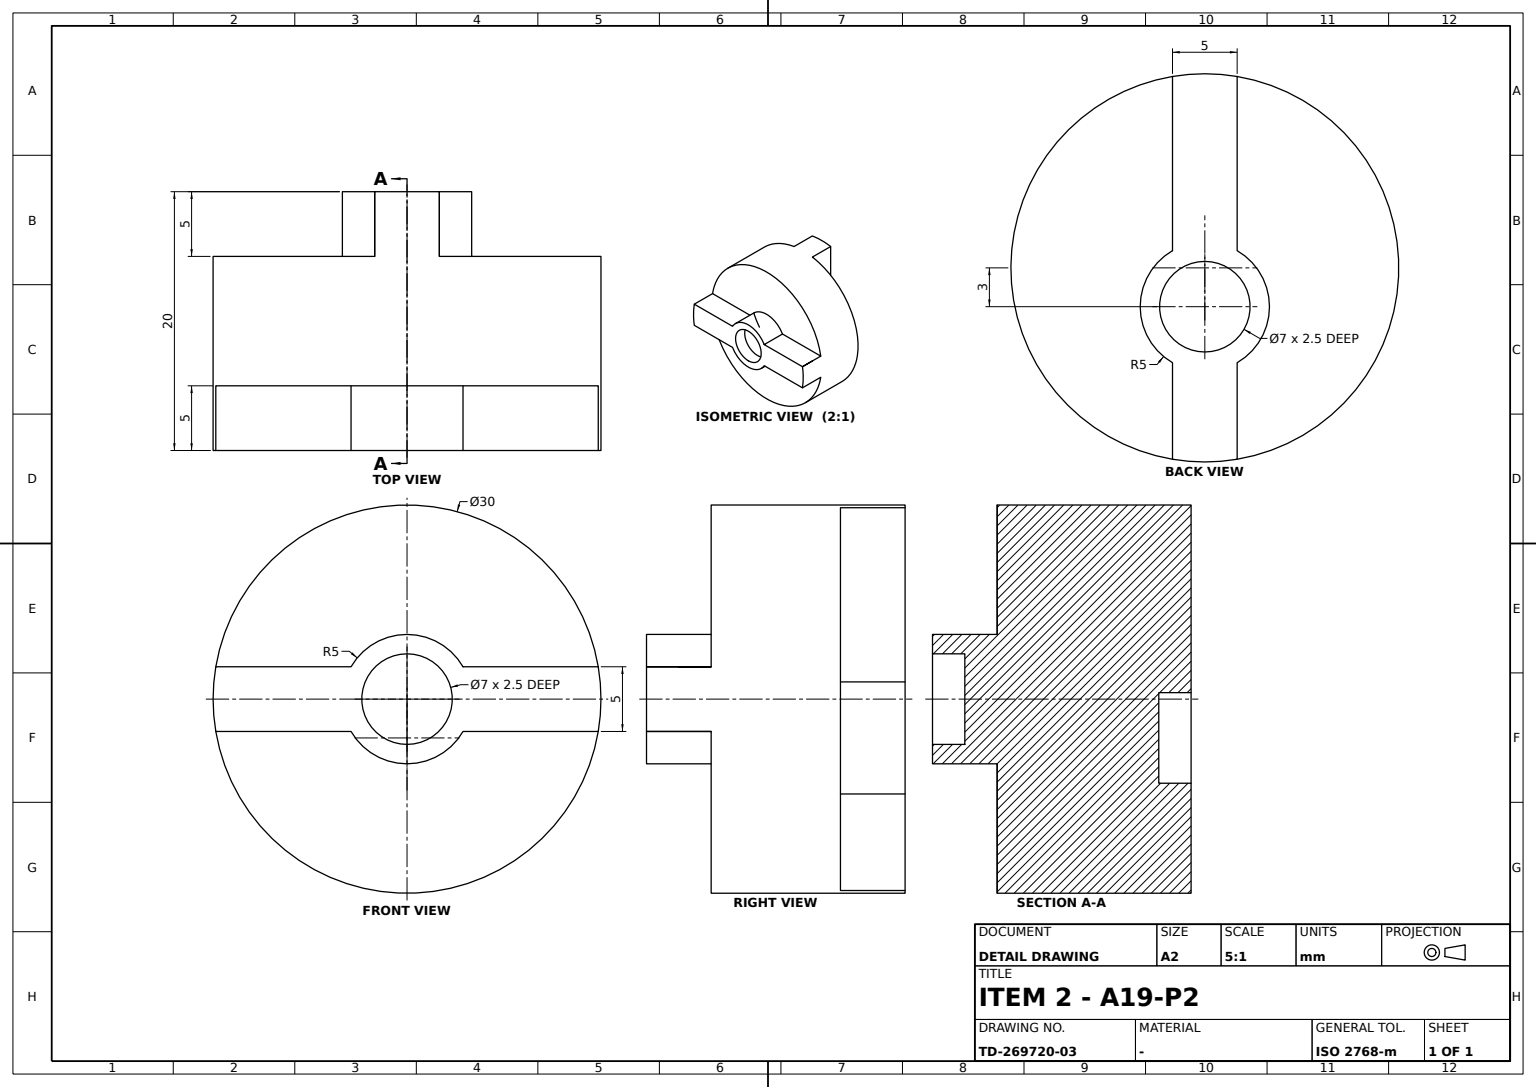
ISO-10303-21;
HEADER;
FILE_DESCRIPTION((''),'2;1');
FILE_NAME('','',(''),(''),'','','');
FILE_SCHEMA(('AUTOMOTIVE_DESIGN'));
ENDSEC;
DATA;
#1=APPLICATION_CONTEXT('');
#2=PRODUCT_CONTEXT('',#1,'mechanical');
#3=PRODUCT('','','',(#2));
#4=PRODUCT_DEFINITION_FORMATION('','',#3);
#5=PRODUCT_DEFINITION_CONTEXT('',#1,'design');
#6=PRODUCT_DEFINITION('','',#4,#5);
#7=PRODUCT_DEFINITION_SHAPE('','',#6);
#8=(LENGTH_UNIT()NAMED_UNIT(*)SI_UNIT(.MILLI.,.METRE.));
#9=(NAMED_UNIT(*)PLANE_ANGLE_UNIT()SI_UNIT($,.RADIAN.));
#10=(NAMED_UNIT(*)SI_UNIT($,.STERADIAN.)SOLID_ANGLE_UNIT());
#11=UNCERTAINTY_MEASURE_WITH_UNIT(LENGTH_MEASURE(0.005),#8,'distance_accuracy_value','');
#12=(GEOMETRIC_REPRESENTATION_CONTEXT(3)GLOBAL_UNCERTAINTY_ASSIGNED_CONTEXT((#11))GLOBAL_UNIT_ASSIGNED_CONTEXT((#8,#9,#10))REPRESENTATION_CONTEXT('',''));
#13=CARTESIAN_POINT('',(-7.5,0.,0.5));
#14=VERTEX_POINT('',#13);
#15=CARTESIAN_POINT('',(-7.5,0.,-3.));
#16=DIRECTION('',(-1.,0.,0.));
#17=DIRECTION('',(0.,0.,1.));
#18=AXIS2_PLACEMENT_3D('',#15,#16,#17);
#19=CIRCLE('',#18,3.5);
#20=EDGE_CURVE('',#14,#14,#19,.T.);
#21=ORIENTED_EDGE('',*,*,#20,.F.);
#22=EDGE_LOOP('',(#21));
#23=FACE_BOUND('',#22,.T.);
#24=CARTESIAN_POINT('',(-10.,0.,0.5));
#25=VERTEX_POINT('',#24);
#26=CARTESIAN_POINT('',(-10.,0.,-3.));
#27=AXIS2_PLACEMENT_3D('',#26,#16,#17);
#28=CIRCLE('',#27,3.5);
#29=EDGE_CURVE('',#25,#25,#28,.T.);
#30=ORIENTED_EDGE('',*,*,#29,.T.);
#31=EDGE_LOOP('',(#30));
#32=FACE_BOUND('',#31,.T.);
#33=CARTESIAN_POINT('',(-8.75,0.,-3.));
#34=DIRECTION('',(0.,-1.,0.));
#35=AXIS2_PLACEMENT_3D('',#33,#16,#34);
#36=CYLINDRICAL_SURFACE('',#35,3.5);
#37=ADVANCED_FACE('',(#23,#32),#36,.F.);
#38=CARTESIAN_POINT('',(7.5,0.,-3.5));
#39=VERTEX_POINT('',#38);
#40=CARTESIAN_POINT('',(7.5,0.,0.));
#41=DIRECTION('',(1.,0.,0.));
#42=DIRECTION('',(0.,0.,-1.));
#43=AXIS2_PLACEMENT_3D('',#40,#41,#42);
#44=CIRCLE('',#43,3.5);
#45=EDGE_CURVE('',#39,#39,#44,.T.);
#46=ORIENTED_EDGE('',*,*,#45,.F.);
#47=EDGE_LOOP('',(#46));
#48=FACE_BOUND('',#47,.T.);
#49=CARTESIAN_POINT('',(10.,0.,-3.5));
#50=VERTEX_POINT('',#49);
#51=CARTESIAN_POINT('',(10.,0.,0.));
#52=AXIS2_PLACEMENT_3D('',#51,#41,#42);
#53=CIRCLE('',#52,3.5);
#54=EDGE_CURVE('',#50,#50,#53,.T.);
#55=ORIENTED_EDGE('',*,*,#54,.T.);
#56=EDGE_LOOP('',(#55));
#57=FACE_BOUND('',#56,.T.);
#58=CARTESIAN_POINT('',(8.75,0.,0.));
#59=DIRECTION('',(0.,1.,0.));
#60=AXIS2_PLACEMENT_3D('',#58,#41,#59);
#61=CYLINDRICAL_SURFACE('',#60,3.5);
#62=ADVANCED_FACE('',(#48,#57),#61,.F.);
#63=CARTESIAN_POINT('',(-5.,-2.5,1.330127));
#64=VERTEX_POINT('',#63);
#65=CARTESIAN_POINT('',(-10.,-2.5,1.330127));
#66=VERTEX_POINT('',#65);
#67=VECTOR('',#16,1000.);
#68=LINE('',#63,#67);
#69=EDGE_CURVE('',#64,#66,#68,.T.);
#70=ORIENTED_EDGE('',*,*,#69,.F.);
#71=CARTESIAN_POINT('',(-5.,-2.5,14.790199));
#72=VERTEX_POINT('',#71);
#73=CARTESIAN_POINT('',(-5.,-2.5,-7.330127));
#74=VECTOR('',#42,1000.);
#75=LINE('',#73,#74);
#76=EDGE_CURVE('',#72,#64,#75,.T.);
#77=ORIENTED_EDGE('',*,*,#76,.F.);
#78=CARTESIAN_POINT('',(-10.,-2.5,14.790199));
#79=VERTEX_POINT('',#78);
#80=VECTOR('',#41,1000.);
#81=LINE('',#71,#80);
#82=EDGE_CURVE('',#72,#79,#81,.F.);
#83=ORIENTED_EDGE('',*,*,#82,.T.);
#84=CARTESIAN_POINT('',(-10.,-2.5,0.));
#85=LINE('',#84,#74);
#86=EDGE_CURVE('',#79,#66,#85,.T.);
#87=ORIENTED_EDGE('',*,*,#86,.T.);
#88=EDGE_LOOP('',(#70,#77,#83,#87));
#89=FACE_BOUND('',#88,.T.);
#90=AXIS2_PLACEMENT_3D('',#73,#59,#42);
#91=PLANE('',#90);
#92=ADVANCED_FACE('',(#89),#91,.F.);
#93=CARTESIAN_POINT('',(-10.,2.5,14.790199));
#94=VERTEX_POINT('',#93);
#95=CARTESIAN_POINT('',(-10.,0.,0.));
#96=AXIS2_PLACEMENT_3D('',#95,#16,#17);
#97=CIRCLE('',#96,15.);
#98=EDGE_CURVE('',#79,#94,#97,.T.);
#99=ORIENTED_EDGE('',*,*,#98,.T.);
#100=CARTESIAN_POINT('',(-10.,2.5,1.330127));
#101=VERTEX_POINT('',#100);
#102=CARTESIAN_POINT('',(-10.,2.5,0.));
#103=VECTOR('',#17,1000.);
#104=LINE('',#102,#103);
#105=EDGE_CURVE('',#101,#94,#104,.T.);
#106=ORIENTED_EDGE('',*,*,#105,.F.);
#107=CARTESIAN_POINT('',(-10.,2.5,-7.330127));
#108=VERTEX_POINT('',#107);
#109=CIRCLE('',#27,5.);
#110=EDGE_CURVE('',#101,#108,#109,.T.);
#111=ORIENTED_EDGE('',*,*,#110,.T.);
#112=CARTESIAN_POINT('',(-10.,2.5,-14.790199));
#113=VERTEX_POINT('',#112);
#114=EDGE_CURVE('',#113,#108,#104,.T.);
#115=ORIENTED_EDGE('',*,*,#114,.F.);
#116=CARTESIAN_POINT('',(-10.,-2.5,-14.790199));
#117=VERTEX_POINT('',#116);
#118=EDGE_CURVE('',#113,#117,#97,.T.);
#119=ORIENTED_EDGE('',*,*,#118,.T.);
#120=CARTESIAN_POINT('',(-10.,-2.5,-7.330127));
#121=VERTEX_POINT('',#120);
#122=EDGE_CURVE('',#121,#117,#85,.T.);
#123=ORIENTED_EDGE('',*,*,#122,.F.);
#124=EDGE_CURVE('',#121,#66,#109,.T.);
#125=ORIENTED_EDGE('',*,*,#124,.T.);
#126=ORIENTED_EDGE('',*,*,#86,.F.);
#127=EDGE_LOOP('',(#99,#106,#111,#115,#119,#123,#125,#126));
#128=FACE_BOUND('',#127,.T.);
#129=ORIENTED_EDGE('',*,*,#29,.F.);
#130=EDGE_LOOP('',(#129));
#131=FACE_BOUND('',#130,.T.);
#132=AXIS2_PLACEMENT_3D('',#95,#16,#34);
#133=PLANE('',#132);
#134=ADVANCED_FACE('',(#128,#131),#133,.T.);
#135=VERTEX_POINT('',#73);
#136=CARTESIAN_POINT('',(-5.,0.,-3.));
#137=AXIS2_PLACEMENT_3D('',#136,#41,#42);
#138=CIRCLE('',#137,5.);
#139=EDGE_CURVE('',#135,#64,#138,.F.);
#140=ORIENTED_EDGE('',*,*,#139,.F.);
#141=CARTESIAN_POINT('',(-5.,-2.5,-14.790199));
#142=VERTEX_POINT('',#141);
#143=EDGE_CURVE('',#135,#142,#75,.T.);
#144=ORIENTED_EDGE('',*,*,#143,.T.);
#145=CARTESIAN_POINT('',(-5.,0.,0.));
#146=AXIS2_PLACEMENT_3D('',#145,#41,#42);
#147=CIRCLE('',#146,15.);
#148=EDGE_CURVE('',#72,#142,#147,.T.);
#149=ORIENTED_EDGE('',*,*,#148,.F.);
#150=ORIENTED_EDGE('',*,*,#76,.T.);
#151=EDGE_LOOP('',(#140,#144,#149,#150));
#152=FACE_BOUND('',#151,.T.);
#153=AXIS2_PLACEMENT_3D('',#145,#41,#59);
#154=PLANE('',#153);
#155=ADVANCED_FACE('',(#152),#154,.F.);
#156=ORIENTED_EDGE('',*,*,#139,.T.);
#157=ORIENTED_EDGE('',*,*,#69,.T.);
#158=ORIENTED_EDGE('',*,*,#124,.F.);
#159=LINE('',#73,#67);
#160=EDGE_CURVE('',#135,#121,#159,.T.);
#161=ORIENTED_EDGE('',*,*,#160,.F.);
#162=EDGE_LOOP('',(#156,#157,#158,#161));
#163=FACE_BOUND('',#162,.T.);
#164=AXIS2_PLACEMENT_3D('',#15,#16,#34);
#165=CYLINDRICAL_SURFACE('',#164,5.);
#166=ADVANCED_FACE('',(#163),#165,.T.);
#167=CARTESIAN_POINT('',(5.,-14.790199,2.5));
#168=VERTEX_POINT('',#167);
#169=CARTESIAN_POINT('',(5.,-4.330127,2.5));
#170=VERTEX_POINT('',#169);
#171=CARTESIAN_POINT('',(5.,0.,2.5));
#172=VECTOR('',#59,1000.);
#173=LINE('',#171,#172);
#174=EDGE_CURVE('',#168,#170,#173,.T.);
#175=ORIENTED_EDGE('',*,*,#174,.F.);
#176=CARTESIAN_POINT('',(10.,-14.790199,2.5));
#177=VERTEX_POINT('',#176);
#178=LINE('',#167,#80);
#179=EDGE_CURVE('',#168,#177,#178,.T.);
#180=ORIENTED_EDGE('',*,*,#179,.T.);
#181=CARTESIAN_POINT('',(10.,-4.330127,2.5));
#182=VERTEX_POINT('',#181);
#183=CARTESIAN_POINT('',(10.,0.,2.5));
#184=LINE('',#183,#172);
#185=EDGE_CURVE('',#177,#182,#184,.T.);
#186=ORIENTED_EDGE('',*,*,#185,.T.);
#187=LINE('',#169,#80);
#188=EDGE_CURVE('',#170,#182,#187,.T.);
#189=ORIENTED_EDGE('',*,*,#188,.F.);
#190=EDGE_LOOP('',(#175,#180,#186,#189));
#191=FACE_BOUND('',#190,.T.);
#192=AXIS2_PLACEMENT_3D('',#167,#42,#59);
#193=PLANE('',#192);
#194=ADVANCED_FACE('',(#191),#193,.F.);
#195=CARTESIAN_POINT('',(-5.,2.5,1.330127));
#196=VERTEX_POINT('',#195);
#197=CARTESIAN_POINT('',(-5.,2.5,14.790199));
#198=VERTEX_POINT('',#197);
#199=CARTESIAN_POINT('',(-5.,2.5,-14.790199));
#200=LINE('',#199,#103);
#201=EDGE_CURVE('',#196,#198,#200,.T.);
#202=ORIENTED_EDGE('',*,*,#201,.T.);
#203=VERTEX_POINT('',#199);
#204=EDGE_CURVE('',#203,#198,#147,.T.);
#205=ORIENTED_EDGE('',*,*,#204,.F.);
#206=CARTESIAN_POINT('',(-5.,2.5,-7.330127));
#207=VERTEX_POINT('',#206);
#208=EDGE_CURVE('',#203,#207,#200,.T.);
#209=ORIENTED_EDGE('',*,*,#208,.T.);
#210=EDGE_CURVE('',#196,#207,#138,.F.);
#211=ORIENTED_EDGE('',*,*,#210,.F.);
#212=EDGE_LOOP('',(#202,#205,#209,#211));
#213=FACE_BOUND('',#212,.T.);
#214=ADVANCED_FACE('',(#213),#154,.F.);
#215=ORIENTED_EDGE('',*,*,#114,.T.);
#216=LINE('',#206,#67);
#217=EDGE_CURVE('',#207,#108,#216,.T.);
#218=ORIENTED_EDGE('',*,*,#217,.F.);
#219=ORIENTED_EDGE('',*,*,#208,.F.);
#220=LINE('',#199,#80);
#221=EDGE_CURVE('',#203,#113,#220,.F.);
#222=ORIENTED_EDGE('',*,*,#221,.T.);
#223=EDGE_LOOP('',(#215,#218,#219,#222));
#224=FACE_BOUND('',#223,.T.);
#225=AXIS2_PLACEMENT_3D('',#199,#34,#17);
#226=PLANE('',#225);
#227=ADVANCED_FACE('',(#224),#226,.F.);
#228=ORIENTED_EDGE('',*,*,#188,.T.);
#229=CARTESIAN_POINT('',(10.,4.330127,2.5));
#230=VERTEX_POINT('',#229);
#231=CIRCLE('',#52,5.);
#232=EDGE_CURVE('',#230,#182,#231,.T.);
#233=ORIENTED_EDGE('',*,*,#232,.F.);
#234=CARTESIAN_POINT('',(5.,4.330127,2.5));
#235=VERTEX_POINT('',#234);
#236=LINE('',#234,#80);
#237=EDGE_CURVE('',#230,#235,#236,.F.);
#238=ORIENTED_EDGE('',*,*,#237,.T.);
#239=CARTESIAN_POINT('',(5.,0.,0.));
#240=AXIS2_PLACEMENT_3D('',#239,#41,#42);
#241=CIRCLE('',#240,5.);
#242=EDGE_CURVE('',#235,#170,#241,.T.);
#243=ORIENTED_EDGE('',*,*,#242,.T.);
#244=EDGE_LOOP('',(#228,#233,#238,#243));
#245=FACE_BOUND('',#244,.T.);
#246=AXIS2_PLACEMENT_3D('',#40,#41,#59);
#247=CYLINDRICAL_SURFACE('',#246,5.);
#248=ADVANCED_FACE('',(#245),#247,.T.);
#249=ORIENTED_EDGE('',*,*,#217,.T.);
#250=ORIENTED_EDGE('',*,*,#110,.F.);
#251=LINE('',#195,#67);
#252=EDGE_CURVE('',#196,#101,#251,.T.);
#253=ORIENTED_EDGE('',*,*,#252,.F.);
#254=ORIENTED_EDGE('',*,*,#210,.T.);
#255=EDGE_LOOP('',(#249,#250,#253,#254));
#256=FACE_BOUND('',#255,.T.);
#257=ADVANCED_FACE('',(#256),#165,.T.);
#258=ORIENTED_EDGE('',*,*,#54,.F.);
#259=EDGE_LOOP('',(#258));
#260=FACE_BOUND('',#259,.T.);
#261=CARTESIAN_POINT('',(10.,-4.330127,-2.5));
#262=VERTEX_POINT('',#261);
#263=CARTESIAN_POINT('',(10.,-14.790199,-2.5));
#264=VERTEX_POINT('',#263);
#265=CARTESIAN_POINT('',(10.,0.,-2.5));
#266=VECTOR('',#34,1000.);
#267=LINE('',#265,#266);
#268=EDGE_CURVE('',#262,#264,#267,.T.);
#269=ORIENTED_EDGE('',*,*,#268,.F.);
#270=CARTESIAN_POINT('',(10.,4.330127,-2.5));
#271=VERTEX_POINT('',#270);
#272=EDGE_CURVE('',#262,#271,#231,.T.);
#273=ORIENTED_EDGE('',*,*,#272,.T.);
#274=CARTESIAN_POINT('',(10.,14.790199,-2.5));
#275=VERTEX_POINT('',#274);
#276=EDGE_CURVE('',#275,#271,#267,.T.);
#277=ORIENTED_EDGE('',*,*,#276,.F.);
#278=CARTESIAN_POINT('',(10.,14.790199,2.5));
#279=VERTEX_POINT('',#278);
#280=CIRCLE('',#52,15.);
#281=EDGE_CURVE('',#275,#279,#280,.T.);
#282=ORIENTED_EDGE('',*,*,#281,.T.);
#283=EDGE_CURVE('',#230,#279,#184,.T.);
#284=ORIENTED_EDGE('',*,*,#283,.F.);
#285=ORIENTED_EDGE('',*,*,#232,.T.);
#286=ORIENTED_EDGE('',*,*,#185,.F.);
#287=EDGE_CURVE('',#177,#264,#280,.T.);
#288=ORIENTED_EDGE('',*,*,#287,.T.);
#289=EDGE_LOOP('',(#269,#273,#277,#282,#284,#285,#286,#288));
#290=FACE_BOUND('',#289,.T.);
#291=AXIS2_PLACEMENT_3D('',#51,#41,#59);
#292=PLANE('',#291);
#293=ADVANCED_FACE('',(#260,#290),#292,.T.);
#294=ORIENTED_EDGE('',*,*,#252,.T.);
#295=ORIENTED_EDGE('',*,*,#105,.T.);
#296=LINE('',#197,#80);
#297=EDGE_CURVE('',#198,#94,#296,.F.);
#298=ORIENTED_EDGE('',*,*,#297,.F.);
#299=ORIENTED_EDGE('',*,*,#201,.F.);
#300=EDGE_LOOP('',(#294,#295,#298,#299));
#301=FACE_BOUND('',#300,.T.);
#302=ADVANCED_FACE('',(#301),#226,.F.);
#303=ORIENTED_EDGE('',*,*,#174,.T.);
#304=ORIENTED_EDGE('',*,*,#242,.F.);
#305=CARTESIAN_POINT('',(5.,14.790199,2.5));
#306=VERTEX_POINT('',#305);
#307=EDGE_CURVE('',#235,#306,#173,.T.);
#308=ORIENTED_EDGE('',*,*,#307,.T.);
#309=CIRCLE('',#240,15.);
#310=EDGE_CURVE('',#306,#168,#309,.T.);
#311=ORIENTED_EDGE('',*,*,#310,.T.);
#312=EDGE_LOOP('',(#303,#304,#308,#311));
#313=FACE_BOUND('',#312,.T.);
#314=AXIS2_PLACEMENT_3D('',#239,#41,#59);
#315=PLANE('',#314);
#316=ADVANCED_FACE('',(#313),#315,.T.);
#317=CARTESIAN_POINT('',(5.,-4.330127,-2.5));
#318=VERTEX_POINT('',#317);
#319=CARTESIAN_POINT('',(5.,4.330127,-2.5));
#320=VERTEX_POINT('',#319);
#321=EDGE_CURVE('',#318,#320,#241,.T.);
#322=ORIENTED_EDGE('',*,*,#321,.T.);
#323=LINE('',#319,#80);
#324=EDGE_CURVE('',#320,#271,#323,.T.);
#325=ORIENTED_EDGE('',*,*,#324,.T.);
#326=ORIENTED_EDGE('',*,*,#272,.F.);
#327=LINE('',#317,#80);
#328=EDGE_CURVE('',#262,#318,#327,.F.);
#329=ORIENTED_EDGE('',*,*,#328,.T.);
#330=EDGE_LOOP('',(#322,#325,#326,#329));
#331=FACE_BOUND('',#330,.T.);
#332=ADVANCED_FACE('',(#331),#247,.T.);
#333=ORIENTED_EDGE('',*,*,#276,.T.);
#334=ORIENTED_EDGE('',*,*,#324,.F.);
#335=CARTESIAN_POINT('',(5.,14.790199,-2.5));
#336=VERTEX_POINT('',#335);
#337=CARTESIAN_POINT('',(5.,0.,-2.5));
#338=LINE('',#337,#266);
#339=EDGE_CURVE('',#336,#320,#338,.T.);
#340=ORIENTED_EDGE('',*,*,#339,.F.);
#341=LINE('',#335,#80);
#342=EDGE_CURVE('',#336,#275,#341,.T.);
#343=ORIENTED_EDGE('',*,*,#342,.T.);
#344=EDGE_LOOP('',(#333,#334,#340,#343));
#345=FACE_BOUND('',#344,.T.);
#346=AXIS2_PLACEMENT_3D('',#335,#17,#34);
#347=PLANE('',#346);
#348=ADVANCED_FACE('',(#345),#347,.F.);
#349=ORIENTED_EDGE('',*,*,#148,.T.);
#350=LINE('',#141,#80);
#351=EDGE_CURVE('',#142,#117,#350,.F.);
#352=ORIENTED_EDGE('',*,*,#351,.T.);
#353=ORIENTED_EDGE('',*,*,#118,.F.);
#354=ORIENTED_EDGE('',*,*,#221,.F.);
#355=ORIENTED_EDGE('',*,*,#204,.T.);
#356=ORIENTED_EDGE('',*,*,#297,.T.);
#357=ORIENTED_EDGE('',*,*,#98,.F.);
#358=ORIENTED_EDGE('',*,*,#82,.F.);
#359=EDGE_LOOP('',(#349,#352,#353,#354,#355,#356,#357,#358));
#360=FACE_BOUND('',#359,.T.);
#361=LINE('',#305,#80);
#362=EDGE_CURVE('',#279,#306,#361,.F.);
#363=ORIENTED_EDGE('',*,*,#362,.F.);
#364=ORIENTED_EDGE('',*,*,#281,.F.);
#365=ORIENTED_EDGE('',*,*,#342,.F.);
#366=CARTESIAN_POINT('',(5.,-14.790199,-2.5));
#367=VERTEX_POINT('',#366);
#368=EDGE_CURVE('',#367,#336,#309,.T.);
#369=ORIENTED_EDGE('',*,*,#368,.F.);
#370=LINE('',#366,#80);
#371=EDGE_CURVE('',#264,#367,#370,.F.);
#372=ORIENTED_EDGE('',*,*,#371,.F.);
#373=ORIENTED_EDGE('',*,*,#287,.F.);
#374=ORIENTED_EDGE('',*,*,#179,.F.);
#375=ORIENTED_EDGE('',*,*,#310,.F.);
#376=EDGE_LOOP('',(#363,#364,#365,#369,#372,#373,#374,#375));
#377=FACE_BOUND('',#376,.T.);
#378=CYLINDRICAL_SURFACE('',#246,15.);
#379=ADVANCED_FACE('',(#360,#377),#378,.T.);
#380=ORIENTED_EDGE('',*,*,#237,.F.);
#381=ORIENTED_EDGE('',*,*,#283,.T.);
#382=ORIENTED_EDGE('',*,*,#362,.T.);
#383=ORIENTED_EDGE('',*,*,#307,.F.);
#384=EDGE_LOOP('',(#380,#381,#382,#383));
#385=FACE_BOUND('',#384,.T.);
#386=ADVANCED_FACE('',(#385),#193,.F.);
#387=ORIENTED_EDGE('',*,*,#20,.T.);
#388=EDGE_LOOP('',(#387));
#389=FACE_BOUND('',#388,.T.);
#390=CARTESIAN_POINT('',(-7.5,0.,0.));
#391=AXIS2_PLACEMENT_3D('',#390,#16,#34);
#392=PLANE('',#391);
#393=ADVANCED_FACE('',(#389),#392,.T.);
#394=ORIENTED_EDGE('',*,*,#45,.T.);
#395=EDGE_LOOP('',(#394));
#396=FACE_BOUND('',#395,.T.);
#397=PLANE('',#246);
#398=ADVANCED_FACE('',(#396),#397,.T.);
#399=ORIENTED_EDGE('',*,*,#371,.T.);
#400=EDGE_CURVE('',#318,#367,#338,.T.);
#401=ORIENTED_EDGE('',*,*,#400,.F.);
#402=ORIENTED_EDGE('',*,*,#328,.F.);
#403=ORIENTED_EDGE('',*,*,#268,.T.);
#404=EDGE_LOOP('',(#399,#401,#402,#403));
#405=FACE_BOUND('',#404,.T.);
#406=ADVANCED_FACE('',(#405),#347,.F.);
#407=ORIENTED_EDGE('',*,*,#143,.F.);
#408=ORIENTED_EDGE('',*,*,#160,.T.);
#409=ORIENTED_EDGE('',*,*,#122,.T.);
#410=ORIENTED_EDGE('',*,*,#351,.F.);
#411=EDGE_LOOP('',(#407,#408,#409,#410));
#412=FACE_BOUND('',#411,.T.);
#413=ADVANCED_FACE('',(#412),#91,.F.);
#414=ORIENTED_EDGE('',*,*,#321,.F.);
#415=ORIENTED_EDGE('',*,*,#400,.T.);
#416=ORIENTED_EDGE('',*,*,#368,.T.);
#417=ORIENTED_EDGE('',*,*,#339,.T.);
#418=EDGE_LOOP('',(#414,#415,#416,#417));
#419=FACE_BOUND('',#418,.T.);
#420=ADVANCED_FACE('',(#419),#315,.T.);
#421=CLOSED_SHELL('',(#37,#62,#92,#134,#155,#166,#194,#214,#227,#248,#257,#293,#302,#316,#332,#348,#379,#386,#393,#398,#406,#413,#420));
#422=MANIFOLD_SOLID_BREP('',#421);
#423=ADVANCED_BREP_SHAPE_REPRESENTATION('',(#422),#12);
#424=SHAPE_DEFINITION_REPRESENTATION(#7,#423);
ENDSEC;
END-ISO-10303-21;
